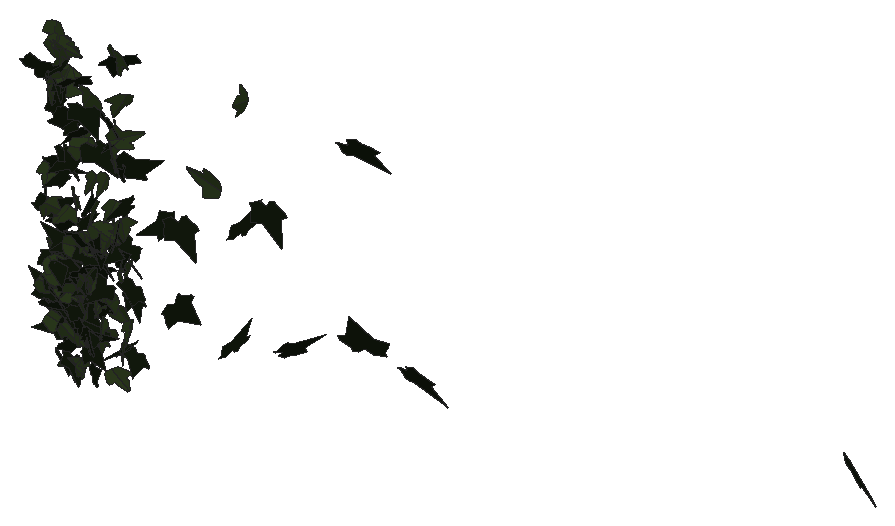
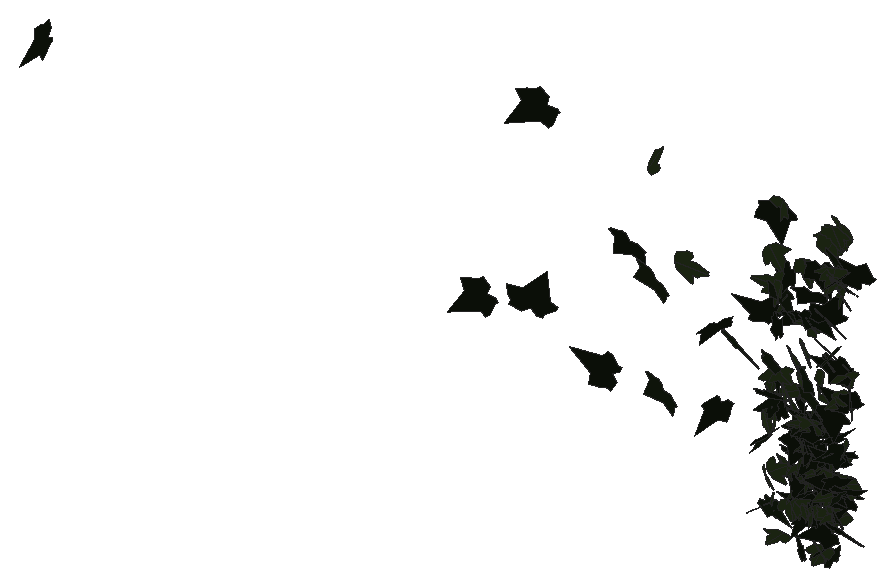
# SketchUp Ruby script. Lengths in inches.
U = 1.inch
M = Sketchup.active_model
def pt(a) = Geom::Point3d.new(a.map { |v| v * U })
def face(e, loops, mat)
  f = e.add_face(loops[0].map { |a| pt(a) })
  loops[1..].each { |l| e.add_face(l.map { |a| pt(a) }).erase! }
  f.material = f.back_material = mat if mat
  f
end
# faces: each face lists its corners as indices into pts; further lists are holes
def faces(e, pts, list, mat = nil) = list.each { |f| face(e, (f[0].is_a?(Array) ? f : [f]).map { |l| l.map { |i| pts[i] } }, mat) }
# xy, xz, yz: faces in a plane at the given z, y or x. An outline is a flat list of corners, or four numbers for a rectangle; further outlines are holes
def ring(l) = l.size == 4 ? [[l[0], l[1]], [l[2], l[1]], [l[2], l[3]], [l[0], l[3]]] : l.each_slice(2).to_a
def flat(e, list, mat, &to3) = list.each { |f| face(e, (f[0].is_a?(Array) ? f : [f]).map { |l| ring(l).map { |u, v| to3.(u, v) } }, mat) }
def xy(e, z, list, mat = nil) = flat(e, list, mat) { |x, y| [x, y, z] }
def xz(e, y, list, mat = nil) = flat(e, list, mat) { |x, z| [x, y, z] }
def yz(e, x, list, mat = nil) = flat(e, list, mat) { |y, z| [x, y, z] }
def lines(e, pts, list) = list.each { |a, b| e.add_line(pt(pts[a]), pt(pts[b])) }
# prism: a flat outline (further loops are holes) pulled along v
def prism(e, loops, v, mat = nil)
  f = face(e, loops, mat); d = Geom::Vector3d.new(v.map { |x| x * U })
  f.pushpull(f.normal.samedirection?(d) ? d.length : -d.length)
end
def box(e, o, s, mat = nil) = prism(e, [[o, [o[0] + s[0], o[1], o[2]], [o[0] + s[0], o[1] + s[1], o[2]], [o[0], o[1] + s[1], o[2]]]], [0, 0, s[2]], mat)
def at(x, y, z, deg = 0) = Geom::Transformation.translation(pt([x, y, z])) * Geom::Transformation.rotation(ORIGIN, Z_AXIS, deg.degrees)
def axes(o, x, y, z) = Geom::Transformation.new([*x, 0, *y, 0, *z, 0, *pt(o).to_a, 1])
def part(name) = M.definitions.add(name)
# library, detail: a bought-in or finely detailed component or shape, given as its bounding box
def library(name, o, s) = part(name).tap { |d| box(d.entities, o, s) }
def detail(e, o, s) = box(e.add_group.entities, o, s)
def put(e, d, t, mat = nil) = e.add_instance(d, t).tap { |i| i.material = mat if mat }
def group(e, t, mat = nil) = e.add_group.tap { |g| g.transformation = t; g.material = mat if mat }.entities
root = M.entities
M.materials.add("1026 AP 7946 SUNNY SIDE UP").color = [254, 231, 186]
M.materials.add("efeu1").color = [18, 25, 13]
M.materials.add("efeu2").color = [43, 57, 29]
c1 = part("ivyleaf_9")
p = [[1.54,2.16,1.25],[1.36,2.04,1.19],[-0.21,0.99,0.68],[-0.71,1.11,0.82],[-0.85,0.86,0.67],[-0.8,0.17,0.21],
  [-0.9,-0.01,0.1],[-0.67,-0.16,-0.02],[-0.08,-0.08,-0.05],[-0.03,-0.6,-0.4],[0.65,-0.88,-0.66],[0.83,-0.6,-0.49],
  [1.29,-0.42,-0.43],[1.8125,-0.07,-0.26],[1.21,0.44,0.15]]
faces(c1.entities,p,[[0,1,2,3,4,5,6,7,8,9,10,11,12,13,14]],"efeu1")
c2 = part("ivyleaf_10")
p = [[0,0.5,-0.03],[-0.0625,2.02,-0.43],[-0.19,2.01,-0.46],[-0.54,1.05,-0.29],[-0.52,0.625,-0.18],[-0.83,0.76,-0.28],
  [-1.16,0.64,-0.33],[-1.15,0.33,-0.24],[-0.77,-0.39,0.02],[-0.3,-0.51,0.16],[0.04,-0.48,0.23],[-0.02,2.01,-0.4375],
  [-0.06,2.01,-0.43],[0.04,-0.49,0.23],[0.67,-0.49,0.14],[1.38,0.36,-0.2],[1.375,0.51,-0.24],[0.81,0.65,-0.19],
  [0.62,0.59,-0.15],[0.6,1.09,-0.28],[0.5,1.23,-0.31]]
faces(c2.entities,p,[[0,1,2,3,4,5,6,7,8,9,10],[11,12,0,13,14,15,16,17,18,19,20]],"efeu2")
put(root,c1,axes([142.79,212.45,277.66],[-0.017,-0.03808,0.31851],[0.43601,-0.14261,-0.00893],[0.22394,0.27477,0.04158]),"1026 AP 7946 SUNNY SIDE UP")
put(root,c1,axes([143.47,212.51,270.16],[-0.39162,-0.1226,-0.06657],[-0.10767,-0.00503,0.28478],[-0.18886,0.25708,-0.02432]),"1026 AP 7946 SUNNY SIDE UP")
put(root,c2,axes([143.18,212.64,274.32],[0.24019,0.22907,-0.10526],[-0.05948,-0.09876,-0.28333],[-0.39073,0.15585,-0.02158]),"1026 AP 7946 SUNNY SIDE UP")
put(root,c1,axes([143.33,212.21,273.04],[0.00078,-0.01663,0.32565],[0.04875,0.31468,0.01884],[-0.49548,0.03093,0.00236]),"1026 AP 7946 SUNNY SIDE UP")
put(root,c2,axes([143.28,212.53,271.78],[-0.14594,0.26324,-0.05837],[0.02491,-0.05607,-0.28786],[-0.42317,-0.09409,0.00319]),"1026 AP 7946 SUNNY SIDE UP")
put(root,c1,axes([143.68,212.71,268.98],[-0.36858,0.10367,0.10381],[-0.16676,0.00552,-0.26151],[-0.15355,-0.25486,0.03483]),"1026 AP 7946 SUNNY SIDE UP")
put(root,c2,axes([143.41,212.43,277.125],[-0.08854,0.2689,0.10331],[-0.07127,0.09101,-0.28139],[-0.44476,-0.06812,0.02452]),"1026 AP 7946 SUNNY SIDE UP")
put(root,c1,axes([143.75,212.58,277.41],[-0.11901,0.19501,0.23284],[-0.30319,0.14468,-0.19524],[-0.3566,-0.1881,0.08829]),"1026 AP 7946 SUNNY SIDE UP")
put(root,c1,axes([143.75,212.26,276.86],[-0.01911,0.16354,0.30569],[-0.13571,0.28468,-0.16413],[-0.51386,-0.08127,0.03198]),"1026 AP 7946 SUNNY SIDE UP")
put(root,c2,axes([143.21,212.4,270.48],[-0.18132,-0.07724,-0.33077],[0.49966,0.06491,-0.13346],[0.13883,-0.3345,0.04835]),"1026 AP 7946 SUNNY SIDE UP")
put(root,c1,axes([143.45,212.82,277.56],[-0.02869,-0.2855,0.06559],[-0.01184,-0.06493,-0.29508],[0.46036,-0.01946,-0.0035]),"1026 AP 7946 SUNNY SIDE UP")
put(root,c1,axes([143.36,212.6875,270.16],[0.14318,-0.24235,0.10163],[0.04992,-0.09492,-0.26724],[0.40922,0.09638,-0.00296]),"1026 AP 7946 SUNNY SIDE UP")
put(root,c1,axes([143.74,212.44,269.3],[0.03492,0.11217,0.28459],[-0.04184,0.27602,-0.1119],[-0.46601,-0.01638,0.03137]),"1026 AP 7946 SUNNY SIDE UP")
put(root,c1,axes([143.8,212.65,271.84],[-0.18733,-0.25661,0.0018],[0.00407,0.00233,0.29147],[-0.4035,0.11915,0.00211]),"1026 AP 7946 SUNNY SIDE UP")
put(root,c1,axes([143.43,212.625,270.66],[-0.00016,-0.19145,-0.21489],[0.06429,0.2053,-0.19396],[0.43925,-0.03012,0.02831]),"1026 AP 7946 SUNNY SIDE UP")
put(root,c2,axes([143.46,212.51,279.34],[0.40057,-0.11864,0.11539],[0.15102,-0.06038,-0.28954],[0.20829,0.27194,-0.01197]),"1026 AP 7946 SUNNY SIDE UP")
put(root,c1,axes([143.32,212.77,271.6],[0.38124,-0.12256,0.0674],[0.07578,-0.0507,-0.27918],[0.20543,0.24614,-0.02209]),"1026 AP 7946 SUNNY SIDE UP")
put(root,c1,axes([143.23,212.65,274.42],[0.30922,0.043,-0.22048],[0.27915,0.13665,0.19691],[0.20038,-0.25672,0.06592]),"1026 AP 7946 SUNNY SIDE UP")
put(root,c1,axes([143.6,212.36,269.89],[0.37069,0.12151,-0.12159],[-0.14063,-0.08387,-0.27188],[-0.22709,0.25027,-0.0301]),"1026 AP 7946 SUNNY SIDE UP")
put(root,c2,axes([143.82,212.49,279.02],[-0.43578,0.0228,0.11948],[-0.18504,-0.07749,-0.27475],[0.01518,-0.29021,0.08092]),"1026 AP 7946 SUNNY SIDE UP")
put(root,c1,axes([143.375,212.3125,273.07],[-0.08738,-0.00176,0.30573],[0.46666,-0.00078,0.05724],[0.00069,0.30193,0.0037]),"1026 AP 7946 SUNNY SIDE UP")
put(root,c1,axes([143.53,212.51,271.42],[-0.12883,-0.26076,-0.10055],[0.06634,0.08738,-0.28074],[0.43192,-0.0912,0.01313]),"1026 AP 7946 SUNNY SIDE UP")
put(root,c2,axes([143.625,212.66,277.66],[-0.24272,-0.23671,-0.12059],[0.12004,0.08817,-0.29022],[0.39651,-0.17159,0.01404]),"1026 AP 7946 SUNNY SIDE UP")
put(root,c2,axes([143.49,212.25,273.3125],[-0.17235,-0.1555,-0.24773],[0.288,0.15865,-0.19147],[0.34463,-0.21035,0.03612]),"1026 AP 7946 SUNNY SIDE UP")
put(root,c2,axes([143.67,212.34,278.8125],[-0.39276,0.16666,-0.00749],[-0.01426,-0.02833,-0.3081],[-0.26198,-0.24831,0.028]),"1026 AP 7946 SUNNY SIDE UP")
put(root,c2,axes([143.51,212.35,271.29],[0.17591,0.2501,0.13659],[0.10474,0.11373,-0.28128],[-0.43154,0.12956,-0.01259]),"1026 AP 7946 SUNNY SIDE UP")
put(root,c2,axes([143.58,212.68,277.81],[0.36733,0.19488,0.028],[0.05897,-0.00441,-0.31217],[-0.30348,0.23502,-0.02676]),"1026 AP 7946 SUNNY SIDE UP")
put(root,c1,axes([143.88,212.51,278.33],[-0.33634,0.18349,-0.11807],[0.12115,-0.08756,-0.29042],[-0.3188,-0.22685,0.0142]),"1026 AP 7946 SUNNY SIDE UP")
put(root,c2,axes([143.48,212.42,269.3],[0.16301,0.14471,0.24774],[0.23718,0.18642,-0.18209],[-0.37085,0.18284,-0.00756]),"1026 AP 7946 SUNNY SIDE UP")
put(root,c1,axes([143.8,212.55,272.79],[0.21795,0.22544,-0.11356],[-0.10267,-0.09071,-0.27306],[-0.38192,0.15304,0.0086]),"1026 AP 7946 SUNNY SIDE UP")
put(root,c1,axes([143.59,212.8125,274.96],[0.17992,-0.25702,-0.04554],[-0.03992,0.03546,-0.28949],[0.40774,0.11688,-0.00825]),"1026 AP 7946 SUNNY SIDE UP")
put(root,c1,axes([143.875,212.7,276.1],[0.25163,0.0774,0.27046],[-0.40384,-0.0612,0.17981],[0.14685,-0.30093,0.03105]),"1026 AP 7946 SUNNY SIDE UP")
put(root,c1,axes([144.05,212.39,274.48],[-0.34502,0.19358,-0.04119],[0.02352,-0.04494,-0.30072],[-0.31027,-0.21866,0.023]),"1026 AP 7946 SUNNY SIDE UP")
put(root,c2,axes([143.9375,212.58,278.44],[-0.21797,-0.17293,-0.24186],[-0.1667,-0.21111,0.2244],[-0.42578,0.17118,0.03596]),"1026 AP 7946 SUNNY SIDE UP")
put(root,c1,axes([143.66,212.68,267.83],[0.0462,-0.15985,0.20972],[0.06495,-0.20029,-0.16858],[0.40291,0.05061,0.00313]),"1026 AP 7946 SUNNY SIDE UP")
put(root,c2,axes([143.93,212.47,273.2],[0.41344,-0.02959,-0.09319],[-0.14518,-0.01679,-0.27141],[0.0353,0.2775,-0.02471]),"1026 AP 7946 SUNNY SIDE UP")
put(root,c1,axes([144.18,212.64,276.17],[-0.2759,0.2117,0.10653],[-0.14249,0.05677,-0.28107],[-0.34107,-0.19496,0.03125]),"1026 AP 7946 SUNNY SIDE UP")
put(root,c2,axes([143.78,212.55,277.3125],[0.49757,-0.09067,-0.01969],[0.04683,0.03705,0.33632],[-0.13779,-0.31481,0.04323]),"1026 AP 7946 SUNNY SIDE UP")
put(root,c2,axes([143.8125,212.5625,269.9375],[0.03027,-0.00525,0.29236],[0.03658,0.28355,0.00544],[-0.44486,0.02296,0.02034]),"1026 AP 7946 SUNNY SIDE UP")
put(root,c2,axes([143.58,212.375,278.9],[-0.20922,-0.0269,-0.30182],[0.46232,-0.01669,-0.13616],[-0.00649,-0.3212,0.03045]),"1026 AP 7946 SUNNY SIDE UP")
put(root,c1,axes([144.13,212.6,275.02],[-0.44502,0.1044,-0.05047],[0.05593,-0.04609,-0.30944],[-0.1729,-0.28361,0.02979]),"1026 AP 7946 SUNNY SIDE UP")
put(root,c1,axes([143.74,212.47,270.98],[-0.15579,0.02466,0.28645],[0.43847,0.01858,0.10083],[-0.01462,0.29446,-0.02861]),"1026 AP 7946 SUNNY SIDE UP")
put(root,c1,axes([143.84,212.52,270.35],[0.07351,0.05354,0.28929],[0.34526,0.175,-0.07108],[-0.28711,0.22415,-0.01141]),"1026 AP 7946 SUNNY SIDE UP")
put(root,c1,axes([143.86,212.55,269.99],[-0.23871,-0.11323,-0.22658],[0.31135,0.0978,-0.19267],[0.23164,-0.24814,0.02548]),"1026 AP 7946 SUNNY SIDE UP")
put(root,c1,axes([144.19,212.59,277.69],[0.0797,0.26807,-0.12929],[-0.05017,-0.12319,-0.28167],[-0.46374,0.0594,0.00825]),"1026 AP 7946 SUNNY SIDE UP")
put(root,c1,axes([143.93,212.52,268.6],[0.04396,0.13563,-0.25577],[0.04762,0.24739,0.14375],[0.44335,-0.04002,0.00992]),"1026 AP 7946 SUNNY SIDE UP")
put(root,c2,axes([144.13,212.59,267.97],[-0.37101,-0.11631,-0.09624],[0.15297,0.01095,-0.26901],[0.17698,-0.25329,0.03077]),"1026 AP 7946 SUNNY SIDE UP")
put(root,c1,axes([144.37,212.8,272.0625],[-0.01439,-0.10933,-0.28787],[-0.05671,-0.27651,0.1113],[-0.46747,0.03691,-0.00464]),"1026 AP 7946 SUNNY SIDE UP")
put(root,c1,axes([144.0625,212.67,268.01],[0.01172,-0.26813,-0.00737],[-0.00283,0.00558,-0.27629],[0.42169,0.00749,-0.00165]),"1026 AP 7946 SUNNY SIDE UP")
put(root,c2,axes([143.83,212.56,270.45],[0.17761,0.11131,0.33774],[0.45258,0.16029,-0.1576],[-0.30088,0.30681,-0.03768]),"1026 AP 7946 SUNNY SIDE UP")
put(root,c2,axes([143.97,212.45,269.1],[-0.24738,0.01025,-0.24776],[0.35179,-0.09998,-0.15571],[-0.13993,-0.26949,0.04655]),"1026 AP 7946 SUNNY SIDE UP")
put(root,c2,axes([144.32,212.43,273.84],[-0.27215,0.21469,0.09247],[-0.11842,0.05257,-0.28268],[-0.34543,-0.18717,0.02405]),"1026 AP 7946 SUNNY SIDE UP")
put(root,c1,axes([144.46,212.3,269.77],[0.12508,-0.02823,-0.28572],[-0.43794,-0.00032,-0.08231],[0.01175,0.28837,-0.02636]),"1026 AP 7946 SUNNY SIDE UP")
put(root,c1,axes([144.48,212.65,276.04],[-0.11317,0.20904,-0.19526],[-0.01678,-0.19866,-0.22133],[-0.44463,-0.04571,0.05805]),"1026 AP 7946 SUNNY SIDE UP")
put(root,c2,axes([144.27,212.55,270.6],[-0.36589,-0.12328,-0.09493],[0.13971,0.02724,-0.27059],[0.19681,-0.24853,0.0156]),"1026 AP 7946 SUNNY SIDE UP")
put(root,c2,axes([144.17,212.59,267.78],[0.00561,-0.08258,-0.27308],[0.23506,-0.22228,0.07224],[-0.36705,-0.14361,0.04209]),"1026 AP 7946 SUNNY SIDE UP")
put(root,c1,axes([144.42,212.62,270.64],[0.27009,-0.2453,-0.03915],[0.05601,-0.01967,0.30784],[-0.38594,-0.17452,0.01728]),"1026 AP 7946 SUNNY SIDE UP")
put(root,c2,axes([144.5,212.4,269.11],[0.00847,0.18569,0.20782],[-0.09646,0.19642,-0.18439],[-0.41895,-0.04147,0.04666]),"1026 AP 7946 SUNNY SIDE UP")
put(root,c2,axes([144.5,212.57,272.34],[0.37087,-0.16888,0.0003],[-0.01959,-0.01955,-0.29801],[0.26483,0.23505,-0.02247]),"1026 AP 7946 SUNNY SIDE UP")
put(root,c2,axes([144.64,212.35,270.16],[-0.26285,0.21841,-0.04227],[-0.0215,0.04269,0.28317],[0.34914,0.16706,-0.01439]),"1026 AP 7946 SUNNY SIDE UP")
put(root,c1,axes([144.47,212.64,271.07],[0.37524,-0.08263,-0.11099],[-0.16428,0.02589,-0.25985],[0.13543,0.26036,-0.0077]),"1026 AP 7946 SUNNY SIDE UP")
put(root,c1,axes([144.82,212.48,273.07],[-0.16204,0.25609,0.08077],[-0.06576,0.06602,-0.28365],[-0.41529,-0.11037,0.0134]),"1026 AP 7946 SUNNY SIDE UP")
put(root,c2,axes([144.35,212.84,275.63],[0.02188,-0.07776,-0.28865],[0.29323,-0.21227,0.0691],[-0.34994,-0.18273,0.03986]),"1026 AP 7946 SUNNY SIDE UP")
put(root,c2,axes([144.61,212.32,271.1],[0.05931,-0.16991,-0.22054],[0.07005,0.21609,-0.1681],[0.4228,-0.01197,0.05879]),"1026 AP 7946 SUNNY SIDE UP")
put(root,c2,axes([144.23,212.42,272.0625],[0.00984,0.01778,0.39579],[0.46134,0.24806,-0.0153],[-0.39077,0.29331,-0.0081]),"1026 AP 7946 SUNNY SIDE UP")
put(root,c2,axes([144.38,212.81,272.27],[0.3323,0.03546,0.17478],[0.26974,-0.00681,-0.21896],[-0.03673,0.27079,-0.02678]),"1026 AP 7946 SUNNY SIDE UP")
put(root,c1,axes([144.64,212.28,271.41],[0.18665,0.25268,0.06323],[0.06817,0.0457,-0.28664],[-0.40261,0.12488,-0.01922]),"1026 AP 7946 SUNNY SIDE UP")
put(root,c1,axes([144.47,212.7,276.76],[-0.18559,-0.17088,-0.21722],[0.27784,0.12479,-0.2063],[0.32235,-0.20594,0.05275]),"1026 AP 7946 SUNNY SIDE UP")
put(root,c1,axes([144.27,212.49,272.19],[0.23412,-0.10276,0.26335],[0.32988,-0.14708,-0.18723],[0.28211,0.25726,0.00039]),"1026 AP 7946 SUNNY SIDE UP")
put(root,c1,axes([144.45,212.67,269.06],[0.00817,-0.0482,-0.27236],[0.41582,-0.04461,0.01348],[-0.07275,-0.26036,0.04649]),"1026 AP 7946 SUNNY SIDE UP")
put(root,c2,axes([144.94,212.45,277.47],[-0.40422,0.0848,0.15538],[-0.23923,0.01606,-0.27725],[-0.12819,-0.29737,0.02744]),"1026 AP 7946 SUNNY SIDE UP")
put(root,c1,axes([144.58,212.3125,270.12],[-0.01407,-0.1083,-0.26034],[0.03875,0.25089,-0.11047],[0.42968,-0.02617,0.00144]),"1026 AP 7946 SUNNY SIDE UP")
put(root,c2,axes([144.47,212.29,275.65],[-0.05095,-0.08162,-0.29103],[0.39886,0.1351,-0.06951],[0.23248,-0.24968,0.05548]),"1026 AP 7946 SUNNY SIDE UP")
put(root,c2,axes([144.71,212.48,269.125],[-0.16574,0.23978,-0.04135],[0.01131,-0.04214,-0.26987],[-0.38247,-0.10515,0.00994]),"1026 AP 7946 SUNNY SIDE UP")
put(root,c1,axes([144.85,212.41,273.51],[0.03857,0.14496,0.2554],[0.01359,0.24751,-0.14903],[-0.45026,0.01989,0.01738]),"1026 AP 7946 SUNNY SIDE UP")
put(root,c1,axes([144.66,212.64,271.9],[-0.0765,-0.25935,-0.07075],[0.03626,0.06399,-0.27125],[0.4197,-0.0528,0.01054]),"1026 AP 7946 SUNNY SIDE UP")
put(root,c2,axes([144.75,212.57,270.11],[-0.04469,0.11803,-0.24837],[-0.01486,-0.2434,-0.1227],[-0.42278,-0.00392,0.03057]),"1026 AP 7946 SUNNY SIDE UP")
put(root,c2,axes([144.95,212.71,269.26],[-0.0443,-0.21651,0.13956],[-0.01766,-0.13635,-0.22565],[0.40223,-0.02983,0.00546]),"1026 AP 7946 SUNNY SIDE UP")
put(root,c2,axes([144.91,212.54,271.37],[0.09315,-0.24997,0.09086],[0.03548,-0.08675,-0.26515],[0.41604,0.06336,0.00227]),"1026 AP 7946 SUNNY SIDE UP")
put(root,c1,axes([145.1,212.65,270.99],[-0.38512,-0.08829,0.08044],[-0.09507,-0.06178,-0.266],[0.15971,-0.24969,0.03564]),"1026 AP 7946 SUNNY SIDE UP")
put(root,c1,axes([144.77,212.76,267.63],[-0.02242,0.07977,0.2585],[0.05407,-0.24812,0.08197],[0.40978,0.0371,0.00333]),"1026 AP 7946 SUNNY SIDE UP")
put(root,c2,axes([144.88,212.39,271.1],[-0.16565,0.2526,-0.05051],[0.01603,-0.05039,-0.28207],[-0.40473,-0.10539,0.00951]),"1026 AP 7946 SUNNY SIDE UP")
put(root,c2,axes([144.98,212.45,274.63],[0.26571,-0.24269,-0.03792],[-0.04084,0.02507,-0.30442],[0.38348,0.17083,-0.00615]),"1026 AP 7946 SUNNY SIDE UP")
put(root,c1,axes([144.94,212.59,271.46],[0.28326,0.20993,-0.0133],[0.00657,-0.02213,-0.28454],[-0.33078,0.17934,-0.01704]),"1026 AP 7946 SUNNY SIDE UP")
put(root,c2,axes([144.96,212.58,271.24],[0.06935,0.2106,-0.17625],[-0.04452,-0.17002,-0.22258],[-0.4255,0.05211,-0.00544]),"1026 AP 7946 SUNNY SIDE UP")
put(root,c1,axes([144.9,212.47,268.72],[0.06296,-0.1662,-0.21259],[-0.10692,0.19428,-0.17446],[0.40149,0.0778,-0.01313]),"1026 AP 7946 SUNNY SIDE UP")
put(root,c2,axes([145.04,212.65,269.15],[-0.38131,0.09872,-0.01536],[0.00759,-0.02898,-0.26867],[-0.15693,-0.24126,0.02432]),"1026 AP 7946 SUNNY SIDE UP")
put(root,c1,axes([145.01,212.57,270.33],[0.3682,0.07562,-0.12914],[-0.17941,-0.05518,-0.25332],[-0.14515,0.26002,-0.01448]),"1026 AP 7946 SUNNY SIDE UP")
put(root,c2,axes([145,212.58,273.65],[0.14945,-0.22219,0.15971],[0.09381,-0.14447,-0.2498],[0.41673,0.1122,-0.00105]),"1026 AP 7946 SUNNY SIDE UP")
put(root,c2,axes([145.03,212.69,270.62],[0.07062,0.235,-0.12464],[-0.02452,-0.12151,-0.24709],[-0.41585,0.04707,-0.00659]),"1026 AP 7946 SUNNY SIDE UP")
put(root,c1,axes([144.73,212.38,269.13],[0.12796,-0.02928,0.262],[0.39583,-0.0403,-0.08794],[0.07459,0.26412,0.01722]),"1026 AP 7946 SUNNY SIDE UP")
put(root,c1,axes([145.22,212.33,272.45],[0.03977,-0.02267,0.29481],[-0.05054,0.28538,0.02787],[-0.44875,-0.03415,0.02299]),"1026 AP 7946 SUNNY SIDE UP")
put(root,c1,axes([145.02,212.68,269.54],[-0.12492,-0.25351,0.05008],[-0.01295,-0.04986,-0.27389],[0.40611,-0.07957,0.00667]),"1026 AP 7946 SUNNY SIDE UP")
put(root,c2,axes([145.05,212.72,270.38],[0.34771,-0.1427,0.06938],[0.06747,-0.05864,-0.27022],[0.23933,0.22385,-0.02463]),"1026 AP 7946 SUNNY SIDE UP")
put(root,c2,axes([145.1,212.85,274.5],[0.31914,-0.20401,0.0385],[0.02256,-0.03997,-0.29613],[0.32568,0.20269,-0.01721]),"1026 AP 7946 SUNNY SIDE UP")
put(root,c2,axes([145.22,212.77,269.28],[-0.29283,-0.18248,0.01562],[-0.00008,-0.02304,-0.26821],[0.28806,-0.18551,0.0158]),"1026 AP 7946 SUNNY SIDE UP")
put(root,c1,axes([145.34,212.58,271.03],[-0.42146,-0.0716,-0.01293],[0.02834,-0.0206,-0.28481],[0.11062,-0.26752,0.0237]),"1026 AP 7946 SUNNY SIDE UP")
put(root,c1,axes([145.0625,212.64,272.13],[0.0252,-0.20225,0.20454],[0.03094,-0.19874,-0.21016],[0.44584,0.02522,0.00302]),"1026 AP 7946 SUNNY SIDE UP")
put(root,c1,axes([145.01,212.57,272.04],[0.25405,-0.22394,0.05492],[0.03392,-0.05167,-0.28449],[0.36084,0.16252,-0.01192]),"1026 AP 7946 SUNNY SIDE UP")
put(root,c2,axes([145.22,212.7,269.66],[-0.02889,0.18792,-0.18852],[-0.01668,-0.18489,-0.19445],[-0.41328,-0.00568,0.02103]),"1026 AP 7946 SUNNY SIDE UP")
put(root,c1,axes([145.02,212.51,275.6875],[-0.0457,-0.19261,-0.23691],[0.22489,0.19301,-0.18492],[0.41311,-0.12638,0.07446]),"1026 AP 7946 SUNNY SIDE UP")
put(root,c2,axes([145.2,212.4,273.03],[-0.24024,-0.08376,-0.24233],[0.38796,-0.01178,-0.16117],[0.05557,-0.27984,0.07753]),"1026 AP 7946 SUNNY SIDE UP")
put(root,c2,axes([145.5,212.86,273.7],[0.19006,0.20644,-0.15944],[-0.13508,-0.13032,-0.2471],[-0.38372,0.14813,0.00802]),"1026 AP 7946 SUNNY SIDE UP")
put(root,c2,axes([145.42,212.53,272.7],[0.31515,-0.18129,0.11176],[0.11224,-0.08413,-0.27856],[0.31355,0.21233,-0.01261]),"1026 AP 7946 SUNNY SIDE UP")
put(root,c2,axes([145.625,212.66,270.59],[0.28955,-0.1876,-0.10663],[-0.12273,0.06686,-0.27029],[0.31289,0.19983,-0.00734]),"1026 AP 7946 SUNNY SIDE UP")
put(root,c2,axes([145.65,212.58,273.12],[0.0708,-0.21186,-0.21469],[-0.08527,0.20015,-0.2218],[0.45809,0.07,-0.00811]),"1026 AP 7946 SUNNY SIDE UP")
put(root,c2,axes([145.93,212.7,270.13],[-0.30574,0.08063,-0.2247],[-0.28946,0.12131,0.21552],[0.22451,0.2662,-0.02813]),"1026 AP 7946 SUNNY SIDE UP")
put(root,c2,axes([145.74,212.6875,276.53],[-0.31027,0.21788,0.06161],[-0.07418,0.03625,-0.30243],[-0.34692,-0.20262,0.00956]),"1026 AP 7946 SUNNY SIDE UP")
put(root,c1,axes([145.65,212.3125,276.94],[0.40487,-0.09459,-0.18111],[-0.27509,0.02947,-0.28099],[0.14965,0.31008,-0.02654]),"1026 AP 7946 SUNNY SIDE UP")
put(root,c1,axes([145.95,212.41,276.28],[-0.15086,0.31467,0.01676],[-0.0341,0.00851,-0.33833],[-0.49414,-0.09665,0.01823]),"1026 AP 7946 SUNNY SIDE UP")
put(root,c2,axes([145.86,212.47,279.23],[-0.44211,0.19251,0.02008],[-0.04793,-0.01206,-0.35],[-0.30027,-0.28151,0.0263]),"1026 AP 7946 SUNNY SIDE UP")
put(root,c2,axes([145.77,212.4,275.98],[-0.13127,0.31208,-0.06959],[0.00403,-0.07099,-0.33284],[-0.50266,-0.08207,0.01551]),"1026 AP 7946 SUNNY SIDE UP")
put(root,c1,axes([145.64,212.85,275.07],[-0.02962,0.01706,0.30536],[0.08523,-0.29172,0.01915],[0.45884,0.05529,0.01615]),"1026 AP 7946 SUNNY SIDE UP")
put(root,c2,axes([145.64,212.71,268.02],[0.24623,0.14761,0.15601],[0.19021,0.09077,-0.22071],[-0.2716,0.19739,-0.01313]),"1026 AP 7946 SUNNY SIDE UP")
put(root,c1,axes([145.95,212.53,279.07],[0.16178,0.29769,-0.12439],[-0.04334,-0.11992,-0.32493],[-0.50427,0.10581,-0.01198]),"1026 AP 7946 SUNNY SIDE UP")
put(root,c1,axes([146.09,212.81,269.03],[-0.25281,0.20787,-0.1129],[0.00892,-0.13066,-0.26184],[-0.37026,-0.14508,0.07078]),"1026 AP 7946 SUNNY SIDE UP")
put(root,c2,axes([146,212.67,277.67],[-0.16781,-0.29273,0.10531],[-0.04076,-0.10107,-0.32142],[0.48671,-0.10939,0.00939]),"1026 AP 7946 SUNNY SIDE UP")
put(root,c1,axes([146.11,212.79,273.97],[-0.37892,0.15233,-0.11329],[0.08728,-0.11455,-0.2872],[-0.28307,-0.23923,0.06309]),"1026 AP 7946 SUNNY SIDE UP")
put(root,c2,axes([146.11,212.37,271.83],[-0.00075,0.03942,0.31816],[-0.28422,0.25115,-0.03187],[-0.39818,-0.17935,0.02215]),"1026 AP 7946 SUNNY SIDE UP")
put(root,c1,axes([145.75,212.6,272.11],[-0.04079,0.03691,0.30025],[0.18906,-0.26539,0.04413],[0.42111,0.12272,0.00927]),"1026 AP 7946 SUNNY SIDE UP")
put(root,c1,axes([145.91,212.5625,273.3],[-0.11111,0.0098,-0.29738],[0.3631,-0.17669,-0.06544],[-0.27296,-0.23903,0.03401]),"1026 AP 7946 SUNNY SIDE UP")
put(root,c2,axes([146.02,212.58,273.39],[0.12826,0.29277,0.07222],[-0.09673,0.08566,-0.30148],[-0.46275,0.06324,0.08303]),"1026 AP 7946 SUNNY SIDE UP")
put(root,c2,axes([145.875,212.8125,269.02],[0.15322,-0.16726,0.19825],[0.21389,-0.14133,-0.19736],[0.34043,0.16408,0.03477]),"1026 AP 7946 SUNNY SIDE UP")
put(root,c1,axes([146.25,212.67,272.6875],[-0.46273,-0.06505,-0.00409],[0.02112,-0.04429,-0.30708],[0.10023,-0.29095,0.04584]),"1026 AP 7946 SUNNY SIDE UP")
put(root,c2,axes([146.15,212.79,271.99],[0.05041,-0.29393,-0.02257],[0.00583,0.02076,-0.30442],[0.46324,0.03173,0.00629]),"1026 AP 7946 SUNNY SIDE UP")
put(root,c1,axes([145.86,212.67,272.42],[0.32281,-0.21362,0.05384],[0.03369,-0.05339,-0.30475],[0.34462,0.20532,-0.02065]),"1026 AP 7946 SUNNY SIDE UP")
put(root,c2,axes([145.97,212.39,276.35],[-0.14985,-0.10848,0.30916],[0.23288,0.2631,0.14767],[-0.44547,0.17404,-0.0268]),"1026 AP 7946 SUNNY SIDE UP")
put(root,c2,axes([146.14,212.76,269.89],[0.27698,-0.16966,0.16326],[0.1658,-0.12012,-0.25239],[0.32639,0.20499,-0.01033]),"1026 AP 7946 SUNNY SIDE UP")
put(root,c1,axes([146.3,212.8,271.1875],[-0.10536,-0.25839,0.11827],[-0.03747,-0.11392,-0.27561],[0.44396,-0.07093,0.00481]),"1026 AP 7946 SUNNY SIDE UP")
put(root,c1,axes([146.32,212.92,268.82],[-0.1157,-0.24528,0.09178],[0.01319,-0.09617,-0.26209],[0.41088,-0.06599,0.03426]),"1026 AP 7946 SUNNY SIDE UP")
put(root,c1,axes([146.3125,212.79,270.99],[0.05359,-0.28259,0.08869],[0.00887,-0.08764,-0.29371],[0.46517,0.03423,-0.00462]),"1026 AP 7946 SUNNY SIDE UP")
put(root,c1,axes([146.21,212.56,275.35],[-0.00683,0.02019,0.33396],[0.50958,-0.01957,0.00562],[0.03125,0.32349,-0.01859]),"1026 AP 7946 SUNNY SIDE UP")
put(root,c1,axes([147.82,212.51,274.02],[-0.41763,0.22265,0.00559],[-0.03109,-0.01713,-0.35615],[-0.34877,-0.26508,0.02506]),"1026 AP 7946 SUNNY SIDE UP")
put(root,c1,axes([148.26,212.38,271.45],[0.04028,-0.12018,-0.38923],[-0.20697,0.35383,-0.1233],[0.58697,0.13301,-0.01676]),"1026 AP 7946 SUNNY SIDE UP")
put(root,c1,axes([148.31,212.46,274.23],[0.05008,-0.33852,-0.17322],[-0.0352,0.16482,-0.34926],[0.59195,0.03844,-0.00611]),"1026 AP 7946 SUNNY SIDE UP")
put(root,c2,axes([149.55,212.55,275.93],[-0.07525,0.0127,-0.39193],[-0.52281,0.18545,0.05054],[0.29166,0.3357,-0.01053]),"1026 AP 7946 SUNNY SIDE UP")
put(root,c1,axes([150.7,212.07,270.94],[-0.34164,0.29143,-0.20747],[-0.15735,0.17815,0.37478],[0.53588,0.23811,-0.02222]),"1026 AP 7946 SUNNY SIDE UP")
put(root,c2,axes([150.53,212.78,279.1],[-0.06654,0.11931,0.35789],[0.19801,-0.32306,0.12847],[0.54149,0.13279,-0.003]),"1026 AP 7946 SUNNY SIDE UP")
put(root,c1,axes([150.77,212.38,274.89],[-0.34566,0.31489,-0.15744],[-0.10783,0.14037,0.39578],[0.54096,0.22919,-0.02171]),"1026 AP 7946 SUNNY SIDE UP")
put(root,c1,axes([151.66,212.49,275.93],[-0.25523,-0.09041,-0.33633],[0.49959,0.08334,-0.18632],[0.18255,-0.35448,0.03966]),"1026 AP 7946 SUNNY SIDE UP")
put(root,c1,axes([152.3125,212.57,271.2],[0.24107,0.34815,-0.08851],[0.0154,0.09148,0.39143],[0.56439,-0.1512,0.02713]),"1026 AP 7946 SUNNY SIDE UP")
put(root,c1,axes([155.375,212.55,272.42],[0.46691,-0.0431,0.27126],[-0.39513,0.08832,0.30707],[-0.14214,-0.38709,0.03744]),"1026 AP 7946 SUNNY SIDE UP")
put(root,c1,axes([155.06,212.3,279.36],[0.60856,0.05862,0.08084],[0.13016,-0.02731,-0.40145],[-0.08155,0.39389,-0.0375]),"1026 AP 7946 SUNNY SIDE UP")
put(root,c1,axes([157.18,212.52,272.17],[0.62602,-0.06365,0.03374],[0.04242,-0.04018,-0.414],[0.10453,0.39748,-0.03404]),"1026 AP 7946 SUNNY SIDE UP")
put(root,c1,axes([174.16,212.42,275.03],[0.53807,-0.25389,-0.15068],[-0.21745,0.05581,-0.4371],[0.4049,0.36736,-0.0345]),"1026 AP 7946 SUNNY SIDE UP")
